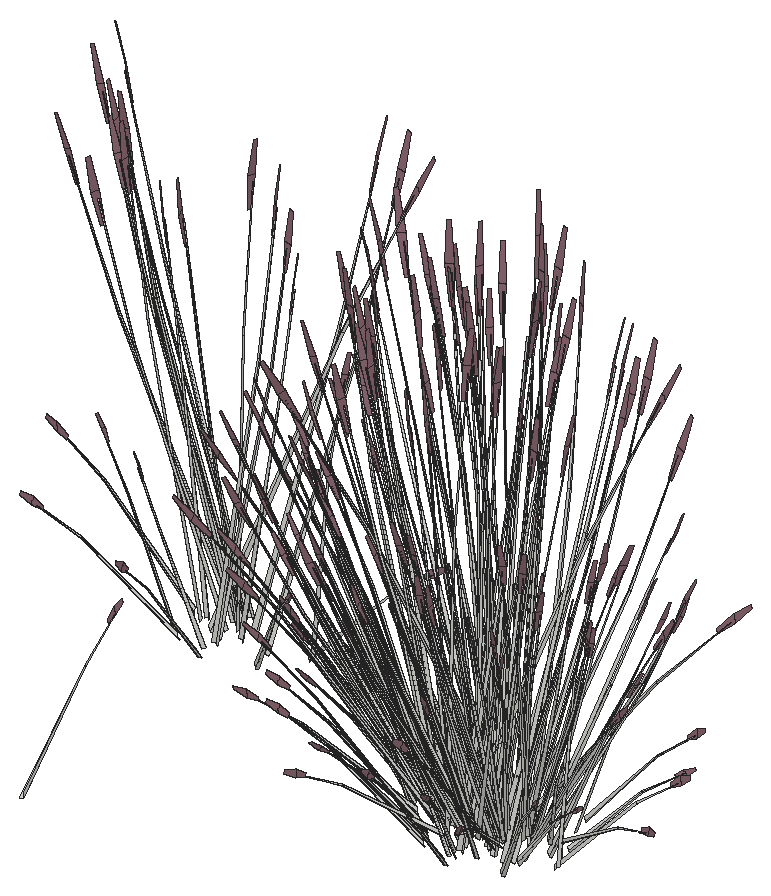
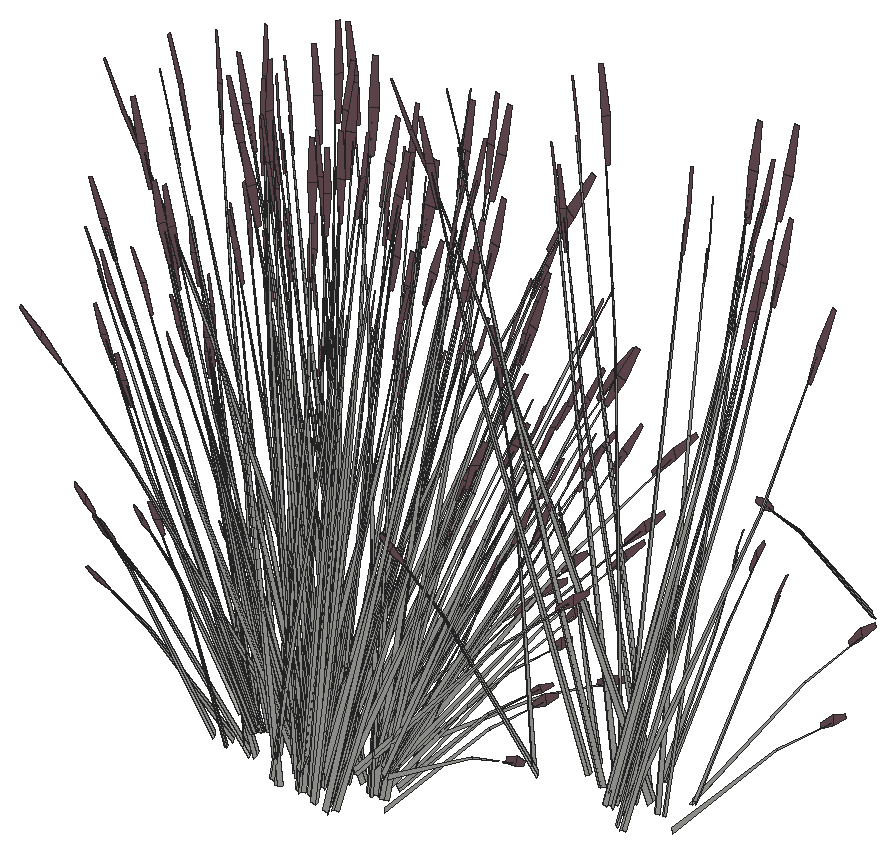
# SketchUp Ruby script. Lengths in inches.
U = 1.inch
M = Sketchup.active_model
def pt(a) = Geom::Point3d.new(a.map { |v| v * U })
def face(e, loops, mat)
  f = e.add_face(loops[0].map { |a| pt(a) })
  loops[1..].each { |l| e.add_face(l.map { |a| pt(a) }).erase! }
  f.material = f.back_material = mat if mat
  f
end
# faces: each face lists its corners as indices into pts; further lists are holes
def faces(e, pts, list, mat = nil) = list.each { |f| face(e, (f[0].is_a?(Array) ? f : [f]).map { |l| l.map { |i| pts[i] } }, mat) }
# xy, xz, yz: faces in a plane at the given z, y or x. An outline is a flat list of corners, or four numbers for a rectangle; further outlines are holes
def ring(l) = l.size == 4 ? [[l[0], l[1]], [l[2], l[1]], [l[2], l[3]], [l[0], l[3]]] : l.each_slice(2).to_a
def flat(e, list, mat, &to3) = list.each { |f| face(e, (f[0].is_a?(Array) ? f : [f]).map { |l| ring(l).map { |u, v| to3.(u, v) } }, mat) }
def xy(e, z, list, mat = nil) = flat(e, list, mat) { |x, y| [x, y, z] }
def xz(e, y, list, mat = nil) = flat(e, list, mat) { |x, z| [x, y, z] }
def yz(e, x, list, mat = nil) = flat(e, list, mat) { |y, z| [x, y, z] }
def lines(e, pts, list) = list.each { |a, b| e.add_line(pt(pts[a]), pt(pts[b])) }
# prism: a flat outline (further loops are holes) pulled along v
def prism(e, loops, v, mat = nil)
  f = face(e, loops, mat); d = Geom::Vector3d.new(v.map { |x| x * U })
  f.pushpull(f.normal.samedirection?(d) ? d.length : -d.length)
end
def box(e, o, s, mat = nil) = prism(e, [[o, [o[0] + s[0], o[1], o[2]], [o[0] + s[0], o[1] + s[1], o[2]], [o[0], o[1] + s[1], o[2]]]], [0, 0, s[2]], mat)
def at(x, y, z, deg = 0) = Geom::Transformation.translation(pt([x, y, z])) * Geom::Transformation.rotation(ORIGIN, Z_AXIS, deg.degrees)
def axes(o, x, y, z) = Geom::Transformation.new([*x, 0, *y, 0, *z, 0, *pt(o).to_a, 1])
def part(name) = M.definitions.add(name)
# library, detail: a bought-in or finely detailed component or shape, given as its bounding box
def library(name, o, s) = part(name).tap { |d| box(d.entities, o, s) }
def detail(e, o, s) = box(e.add_group.entities, o, s)
def put(e, d, t, mat = nil) = e.add_instance(d, t).tap { |i| i.material = mat if mat }
def group(e, t, mat = nil) = e.add_group.tap { |g| g.transformation = t; g.material = mat if mat }.entities
root = M.entities
M.materials.add("LightPink_Translucent").color = [144, 107, 117]
c1 = part("blade")
p = [[2.15,0.21,22],[0,0.17,0],[0.09,0.45,0],[2.18,0.31,22],[2.29,0.31,22],[0.38,0.45,0],
  [2.48,0.24,33],[2.49,0.24,33],[2.48,0.22,33]]
faces(c1.entities,p,[[0,1,2,3],[4,5,2,3],[6,3,4,7],[8,0,3,6]])
c2 = part("seeds")
p = [[0.3,-0.1,1.38],[-0.01,-0.03,1.59],[-0.01,-0.03,0.03],[0.14,-0.07,-0.07],[0.29,-0.03,3],[0.15,0.01,3.11]]
faces(c2.entities,p,[[0,1,2,3],[1,0,4,5]],"LightPink_Translucent")
c3 = part("blade with seeds")
put(c3.entities,c1,at(0,0,0))
put(c3.entities,c2,axes([2.4,0.25,30.99],[1.5799,-0.05474,1.17369],[-0.12525,1.92788,0.29478],[-0.07173,-0.02425,1.56792]))
put(root,c3,axes([47.84,476.29,43.49],[0.19833,-0.05635,1.76342],[1.19302,0.31018,-0.26939],[0.03489,0.3496,0.30037]))
put(root,c3,axes([72.59,505.67,36.13],[0.28013,0.33252,1.71376],[-1.29445,0.27994,0.13857],[-0.29256,-0.52202,0.73262]))
put(root,c3,axes([74.73,503.46,36.97],[-0.18744,-0.14521,1.74944],[-1.25089,0.09206,-0.27667],[-0.19964,-0.34731,0.14031]))
put(root,c3,axes([77.625,505.1875,34.85],[-0.34835,0.20963,1.43002],[-1.04325,-0.36691,-0.30754],[0.19338,-0.4563,0.61141]))
put(root,c3,axes([76.04,505.92,37.24],[-0.5849,-0.8421,-0.71045],[1.20401,-0.4693,0.08574],[-0.13677,-0.40688,1.00501]))
put(root,c3,axes([72.23,504.79,34.85],[-0.07421,0.33879,1.43002],[-1.08488,0.28361,-0.30754],[-0.25359,-0.4379,0.61141]))
put(root,c3,axes([75.03,504.05,33.75],[-0.20555,0.03731,1.76342],[-1.13672,-0.42002,-0.26939],[0.01907,-0.35034,0.30037]))
put(root,c3,axes([78.47,506.74,37.24],[0.03189,-0.95798,-0.71045],[1.34277,0.06434,0.08574],[0.14171,-0.40585,1.00501]))
put(root,c3,axes([80.35,505.24,36.97],[-0.01183,-0.20612,1.74944],[-0.99913,-0.59572,-0.27667],[0.15447,-0.36112,0.14031]))
put(root,c3,axes([76.15,505.2,36.78],[0.36946,-0.79643,-0.35414],[1.07787,0.23229,0.4572],[-0.09883,-0.32066,0.87481]))
put(root,c3,axes([76.96,506.25,36.13],[-0.22818,0.35597,1.71376],[-0.95725,-0.73667,0.13857],[0.43183,-0.45914,0.73262]))
put(root,c3,axes([80.08,504.5,36.96],[-0.12446,0.07911,1.77383],[-1.21937,-0.26689,-0.16761],[-0.04414,-0.34521,0.31391]))
put(root,c3,axes([75.6,505.75,36.94],[-1.20468,-0.25962,-0.51099],[0.41292,-0.89013,-0.3958],[-0.11046,-0.35838,0.97773]))
put(root,c3,axes([76.34,503.52,35.02],[0.15721,0.60392,1.1486],[-0.87211,-0.33448,0.84392],[0.09385,-0.30923,0.25299]))
put(root,c3,axes([78.2,506.42,36.94],[-0.87728,-0.69587,-0.51099],[0.92674,-0.60943,-0.3958],[0.13348,-0.35356,0.97773]))
put(root,c3,axes([73.44,502.99,36.96],[-0.02286,0.12414,1.77383],[-1.12758,0.45052,-0.16761],[-0.33182,-0.23029,0.31391]))
put(root,c3,axes([73.2,505.19,37.35],[1.36515,-0.26619,0.53763],[0.23692,1.04421,0.4433],[-0.32106,-0.30775,1.11249]))
put(root,c3,axes([76.28,505.39,36.99],[1.20755,0.27075,0.48003],[-0.41292,0.89013,0.3958],[-0.07257,-0.35005,0.9933]))
put(root,c3,axes([76.63,505.7,37.29],[-1.19922,0.48218,-0.1216],[-0.58932,-0.85579,-0.67495],[-0.15822,-0.36063,1.02557]))
put(root,c3,axes([79.12,506.79,37.29],[-1.34686,-0.05131,-0.1216],[0.03681,-0.97156,-0.67495],[0.09356,-0.37418,1.02557]))
put(root,c3,axes([79.03,506.16,36.78],[0.82919,-0.54528,-0.35414],[0.78493,0.62262,0.4572],[0.11943,-0.31634,0.87481]))
put(root,c3,axes([71.86,504.24,35.02],[0.63926,0.36046,1.1486],[-0.93099,0.21668,0.84392],[-0.1992,-0.27702,0.25299]))
put(root,c3,axes([76.6,505.32,36.98],[0.90301,-0.35198,0.0643],[0.44199,0.64184,0.50621],[-0.08721,-0.28293,0.77189]))
put(root,c3,axes([73.4,506.15,37.24],[-1.04497,-0.50058,-0.71045],[0.74264,-0.8772,0.08574],[-0.3786,-0.29889,1.00501]))
put(root,c3,axes([73.04,505.49,36.78],[-0.18927,-0.83419,-0.35414],[1.08199,-0.22027,0.4572],[-0.29062,-0.23905,0.87481]))
put(root,c3,axes([45.08,506.35,43.49],[-0.20555,0.03731,1.76342],[-1.13672,-0.42002,-0.26939],[0.01907,-0.35034,0.30037]))
put(root,c3,axes([73.51,505.42,36.98],[0.55698,-0.6579,0.0643],[0.79316,0.38303,0.50621],[-0.25643,-0.21093,0.77189]))
put(root,c3,axes([71.35,505.33,33.75],[-0.11871,0.13643,1.76342],[-1.19964,0.29415,-0.26939],[-0.2898,-0.26759,0.30037]))
put(root,c3,axes([73.33,509.08,34.35],[-0.50328,-1.06202,-0.69835],[1.44974,-0.38248,-0.18329],[-0.05563,-0.35963,1.54149]))
put(root,c3,axes([70.71,506.71,36.13],[0.45521,0.17844,1.71376],[-0.94204,0.74856,0.13857],[-0.58713,-0.33769,0.73262]))
put(root,c3,axes([80.0625,505.83,33.75],[-0.18342,-0.08159,1.76342],[-0.47115,-0.9115,-0.26939],[0.31784,-0.24736,0.30037]))
put(root,c3,axes([76.27,506.04,37.31],[-0.36946,0.79643,0.35414],[-1.07787,-0.23229,-0.4572],[-0.09883,-0.32066,0.87481]))
put(root,c3,axes([72.91,506.18,36.94],[-1.20928,0.24619,-0.51099],[-0.21154,-0.93233,-0.3958],[-0.32481,-0.26718,0.97773]))
put(root,c3,axes([79.02,506.375,36.99],[0.87265,0.70663,0.48003],[-0.92674,0.60943,0.3958],[0.16097,-0.33153,0.9933]))
put(root,c3,axes([73.76,505.35,37.68],[-0.81789,0.99285,-0.13619],[-1.18445,-0.572,-0.75594],[-0.41173,-0.28051,1.14864]))
put(root,c3,axes([79.35,506.44,36.98],[1.00708,0.04826,0.0643],[-0.02761,0.72867,0.50621],[0.10538,-0.27912,0.77189]))
put(root,c3,axes([78.59,506.9375,37.31],[-0.82919,0.54528,0.35414],[-0.78493,-0.62262,-0.4572],[0.11943,-0.31634,0.87481]))
put(root,c3,axes([80.06,508.41,37.24],[0.64013,-0.81717,-0.71045],[1.12174,0.58074,0.08574],[0.38221,-0.29607,1.00501]))
put(root,c3,axes([73.14,506.03,34.63],[-0.7662,-1.03778,0],[1.28187,-0.57875,-0.51607],[0.29196,-0.13181,1.63711]))
put(root,c3,axes([80.02,508.02,36.94],[-0.31482,-0.94565,-0.51099],[1.19224,-0.16542,-0.3958],[0.34166,-0.254,0.97773]))
put(root,c3,axes([74.82,504.78,34.38],[-0.84686,0.59414,-0.03893],[-0.77596,-0.65071,-0.17649],[-0.05463,-0.18438,0.58215]))
put(root,c3,axes([70.625,505.0625,36.97],[-0.26368,-0.00731,1.74944],[-0.83946,0.73103,-0.27667],[-0.44791,-0.14937,0.14031]))
put(root,c3,axes([80.59,508.7,37.29],[-1.1336,-0.57106,-0.1216],[0.65308,-0.827,-0.67495],[0.32027,-0.28747,1.02557]))
put(root,c3,axes([75.9,511.82,35.58],[1.05902,0.41762,1.51261],[-1.03748,0.89969,0.59816],[-0.46471,-0.53324,1.26806]))
put(root,c3,axes([41.41,507.64,43.49],[-0.11871,0.13643,1.76342],[-1.19964,0.29415,-0.26939],[-0.2898,-0.26759,0.30037]))
put(root,c3,axes([73.68,506.17,37.31],[0.18927,0.83419,0.35414],[-1.08199,0.22027,-0.4572],[-0.29062,-0.23905,0.87481]))
put(root,c3,axes([70.37,508.93,34.27],[0,-1.03566,-0.49651],[1.37109,0,0],[0,-0.23588,1.57504]))
put(root,c3,axes([74.18,505.86,34.27],[1.14694,-0.51783,-0.49651],[0.68554,0.92854,0],[0.26122,-0.11794,1.57504]))
put(root,c3,axes([80.98,507.65,34.85],[-0.4378,-0.03068,1.43002],[-0.44851,-0.8229,-0.30754],[0.53783,-0.23279,0.61141]))
put(root,c3,axes([70.43,506.72,37.35],[1.01205,-0.7643,0.53763],[0.87284,0.81167,0.4433],[-0.47482,-0.14098,1.11249]))
put(root,c3,axes([83.38,508.45,36.96],[-0.16006,-0.00787,1.77383],[-0.66468,-0.8428,-0.16761],[0.26693,-0.27711,0.31391]))
put(root,c3,axes([43.39,511.39,44.1],[-0.50328,-1.06202,-0.69835],[1.44974,-0.38248,-0.18329],[-0.05563,-0.35963,1.54149]))
put(root,c3,axes([50.11,508.14,43.49],[-0.18342,-0.08159,1.76342],[-0.47115,-0.9115,-0.26939],[0.31784,-0.24736,0.30037]))
put(root,c3,axes([75.54,507.99,34.3125],[0.82544,-0.77843,-0.62353],[1.0254,0.70586,-0.16365],[0.33076,-0.19418,1.37633]))
put(root,c3,axes([81.49,506.14,35.02],[-0.40819,0.5272,1.1486],[-0.35086,-0.70831,0.84392],[0.33713,-0.17749,0.25299]))
put(root,c3,axes([80.9,508.12,36.78],[1.06674,-0.14801,-0.35414],[0.28168,0.84611,0.4572],[0.30569,-0.22726,0.87481]))
put(root,c3,axes([70.89,506.71,36.98],[0.06171,-0.78753,0.0643],[0.9318,0.02159,0.50621],[-0.35694,-0.08241,0.77189]))
put(root,c3,axes([74.1,509.35,34.47],[0.59459,-0.93321,-0.44739],[1.23546,0.44912,0.21531],[0,-0.21512,1.43643]))
put(root,c3,axes([70.54,506.96,36.78],[-0.69728,-0.64842,-0.35414],[0.79619,-0.61382,0.4572],[-0.40453,-0.09339,0.87481]))
put(root,c3,axes([74.64,508.89,34.92],[-0.1428,-1.18174,-0.29095],[1.48733,-0.07145,-0.50002],[0.26191,-0.15741,1.59708]))
put(root,c3,axes([70.95,508.95,34.28],[0.85545,-0.64616,-0.30978],[0.85545,0.64616,0.30978],[0,-0.20813,1.38974]))
put(root,c3,axes([44.87,507.08,44.13],[-0.84686,0.59414,-0.03893],[-0.77596,-0.65071,-0.17649],[-0.05463,-0.18438,0.58215]))
put(root,c3,axes([70.61,505.86,34.38],[-0.35352,0.84566,-0.03893],[-1.08806,-0.26014,-0.17649],[-0.1652,-0.13832,0.58215]))
put(root,c3,axes([80.03,508.62,37.31],[-1.06674,0.14801,0.35414],[-0.28168,-0.84611,-0.4572],[0.30569,-0.22726,0.87481]))
put(root,c3,axes([73.95,510.13,34.92],[-1.38012,-0.49416,-0.29095],[0.66454,-1.04299,-0.50002],[-0.04337,-0.25608,1.59708]))
put(root,c3,axes([70.02,509.72,34.63],[-1.53239,0,0],[0,-1.1575,-0.51607],[0,-0.26363,1.63711]))
put(root,c3,axes([70.29,507.65,34.85],[0.23927,0.28834,1.43002],[-0.55135,0.78376,-0.30754],[-0.56612,-0.18733,0.61141]))
put(root,c3,axes([74.45,506.27,34.28],[1.14332,0.25625,-0.30978],[-0.28787,0.90242,0.30978],[0.23049,-0.10406,1.38974]))
put(root,c3,axes([71.27,507.39,37.24],[-1.22504,-0.02494,-0.71045],[0.08228,-1.05005,0.08574],[-0.51899,-0.11081,1.00501]))
put(root,c3,axes([40.42,511.24,44.02],[0,-1.03566,-0.49651],[1.37109,0,0],[0,-0.23588,1.57504]))
put(root,c3,axes([44.23,508.17,44.02],[1.14694,-0.51783,-0.49651],[0.68554,0.92854,0],[0.26122,-0.11794,1.57504]))
put(root,c3,axes([81,508.49,36.98],[0.8413,0.43556,0.0643],[-0.48981,0.62025,0.50621],[0.26973,-0.20053,0.77189]))
put(root,c3,axes([80.77,508.31,36.99],[0.30393,0.95317,0.48003],[-1.19224,0.16542,0.3958],[0.35138,-0.22417,0.9933]))
put(root,c3,axes([83.98,509.46,36.97],[0.17006,-0.15775,1.74944],[-0.21766,-0.96766,-0.27667],[0.42669,-0.18347,0.14031]))
put(root,c3,axes([45.59,510.3,44.06],[0.82544,-0.77843,-0.62353],[1.0254,0.70586,-0.16365],[0.33076,-0.19418,1.37633]))
put(root,c3,axes([71.21,509.41,34.58],[-1.1399,0.87071,0.30756],[-1.1406,-0.86155,-0.36492],[-0.03981,-0.24727,1.64885]))
put(root,c3,axes([69.61,505.68,36.96],[0.09085,0.10335,1.77383],[-0.43798,0.92907,-0.16761],[-0.44357,0.00672,0.31391]))
put(root,c3,axes([74.84,509.82,34.6875],[1.3808,0.50196,0.24065],[-0.66454,1.04299,0.50002],[0,-0.24043,1.60543]))
put(root,c3,axes([74.3,511.23,34.69],[0.32481,-1.2272,-0.23429],[1.54007,0.21392,0.51271],[-0.26911,-0.16947,1.5644]))
put(root,c3,axes([44.15,511.66,44.21],[0.59459,-0.93321,-0.44739],[1.23546,0.44912,0.21531],[0,-0.21512,1.43643]))
put(root,c3,axes([70.87,507.6,36.94],[-0.88986,0.68603,-0.51099],[-0.77932,-0.72471,-0.3958],[-0.45212,-0.10438,0.97773]))
put(root,c3,axes([44.69,511.2,44.67],[-0.1428,-1.18174,-0.29095],[1.48733,-0.07145,-0.50002],[0.26191,-0.15741,1.59708]))
put(root,c3,axes([71.53,507.3,37.31],[0.69728,0.64842,0.35414],[-0.79619,0.61382,-0.4572],[-0.40453,-0.09339,0.87481]))
put(root,c3,axes([41.01,511.26,44.03],[0.85545,-0.64616,-0.30978],[0.85545,0.64616,0.30978],[0,-0.20813,1.38974]))
put(root,c3,axes([68.86,508.51,35.02],[0.78239,-0.07411,1.1486],[-0.49629,0.65296,0.84392],[-0.38663,-0.09795,0.25299]))
put(root,c3,axes([40.66,508.16,44.13],[-0.35352,0.84566,-0.03893],[-1.08806,-0.26014,-0.17649],[-0.1652,-0.13832,0.58215]))
put(root,c3,axes([44,512.4375,44.67],[-1.38012,-0.49416,-0.29095],[0.66454,-1.04299,-0.50002],[-0.04337,-0.25608,1.59708]))
put(root,c3,axes([74.39,509.12,34.97],[-1.33077,0.06393,0.44739],[-0.12035,-1.06125,-0.21531],[0.23824,-0.10756,1.43643]))
put(root,c3,axes([71.33,506.89,37.29],[-0.06562,1.05324,-0.1216],[-1.2424,-0.02879,-0.67495],[-0.4785,-0.07316,1.02557]))
put(root,c3,axes([70.95,509.89,34.73],[0,1.03566,0.49651],[-1.37109,0,0],[0,-0.23588,1.57504]))
put(root,c3,axes([80.63,510.93,37.29],[-0.6166,-0.93779,-0.1216],[1.09436,-0.46085,-0.67495],[0.46117,-0.12373,1.02557]))
put(root,c3,axes([44.5,508.58,44.03],[1.14332,0.25625,-0.30978],[-0.28787,0.90242,0.30978],[0.23049,-0.10406,1.38974]))
put(root,c3,axes([80.58,510.12,36.94],[0.332,-0.94205,-0.51099],[1.13828,0.3229,-0.3958],[0.45829,-0.08638,0.97773]))
put(root,c3,axes([78.78,506.29,34.63],[0.7662,-1.03778,0],[1.28187,0.57875,-0.51607],[0.29196,0.13181,1.63711]))
put(root,c3,axes([69.75,508.34,36.13],[0.50831,-0.02346,1.71376],[-0.33721,1.01661,0.13857],[-0.72439,-0.06288,0.73262]))
put(root,c3,axes([74.19,510.73,34.47],[-0.73619,-0.86927,-0.44739],[1.11511,-0.61213,0.21531],[-0.23824,-0.10756,1.43643]))
put(root,c3,axes([74.34,509.5,34.62],[0.53281,1.15808,0.45755],[-1.52239,0.4027,0.17955],[0.01861,-0.2128,1.58856]))
put(root,c3,axes([81.79,510.39,34.24],[-0.7893,0.12429,1.41583],[-0.12563,-0.9893,0.08104],[0.55282,-0.14974,0.80566]))
put(root,c3,axes([83.23,509.51,34.52],[-0.75977,-0.66224,-0.06488],[0.83212,-0.6068,-0.29416],[0.23578,-0.04272,0.97024]))
put(root,c3,axes([74.08,510.41,34.97],[-0.59459,0.93321,0.44739],[-1.23546,-0.44912,-0.21531],[0,-0.21512,1.43643]))
put(root,c3,axes([76.26,509.6,34.46],[0,-1.19833,0],[1.53239,0,0],[0,0,1.79456]))
put(root,c3,axes([78.12,506.83,34.73],[-1.14694,-0.51783,0.49651],[0.68554,-0.92854,0],[0.26122,0.11794,1.57504]))
put(root,c3,axes([80.36,510.47,37.24],[1.07686,-0.45739,-0.71045],[0.60013,0.94154,0.08574],[0.52031,-0.10696,1.00501]))
put(root,c3,axes([73.53,511.0625,34.3125],[-1.27479,-0.1698,-0.62353],[0.26901,-1.04736,-0.16365],[-0.38043,-0.12691,1.37633]))
put(root,c3,axes([75.53,508.84,34.62],[-1.01611,0.93987,0.45755],[-1.20717,-0.82966,0.17955],[0.24496,-0.0938,1.58856]))
put(root,c3,axes([76.64,510.53,34.55],[-1.1399,-0.8914,-0.06131],[1.1406,-0.89194,0],[-0.03981,-0.03113,1.75571]))
put(root,c3,axes([73.77,507.3,34.73],[-0.35402,1.02926,0.17642],[-1.29548,-0.29127,0.35086],[0.22379,-0.00501,1.60407]))
put(root,c3,axes([80.2,510.65,37.31],[-1.01846,-0.28891,0.35414],[0.29705,-0.84289,-0.4572],[0.41005,-0.07729,0.87481]))
put(root,c3,axes([44.35,513.53,44.4375],[0.32481,-1.2272,-0.23429],[1.54007,0.21392,0.51271],[-0.26911,-0.16947,1.5644]))
put(root,c3,axes([69.54,509.11,36.99],[0.34623,-0.9443,0.48003],[1.13828,0.3229,0.3958],[-0.44763,0.05675,0.9933]))
put(root,c3,axes([73.23,508.125,33.85],[-1.20625,0.41464,1.28929],[-0.38394,-1.1897,0.50096],[0.74071,0.01979,1.46642]))
put(root,c3,axes([76.48,508.44,34.87],[0.23642,-0.92427,0.1448],[1.15506,0.16044,-0.41347],[0.21021,0.09491,1.26744]))
put(root,c3,axes([69.46,508.86,36.98],[-0.4501,-0.70615,0.0643],[0.82077,-0.34564,0.50621],[-0.36181,0.0682,0.77189]))
put(root,c3,axes([74.48,510.64,34.62],[1.54892,0.2182,0.45755],[-0.31522,1.23236,0.17955],[-0.22636,-0.119,1.58856]))
put(root,c3,axes([82.66,509.74,33.75],[-0.06405,-0.15723,1.76342],[0.44421,-0.91974,-0.26939],[0.4481,-0.01323,0.30037]))
put(root,c3,axes([69.43,509.58,33.75],[0.03108,0.16322,1.76342],[-0.62654,0.85237,-0.26939],[-0.44504,-0.04296,0.30037]))
put(root,c3,axes([75.98,508.68,34.97],[-0.73619,-0.86927,0.44739],[1.11511,-0.61213,-0.21531],[0.23824,0.10756,1.43643]))
put(root,c3,axes([72.18,512.66,34.28],[-0.28787,-0.90242,-0.30978],[1.14332,-0.25625,0.30978],[-0.23049,-0.10406,1.38974]))
put(root,c3,axes([44.24,513.03,44.21],[-0.73619,-0.86927,-0.44739],[1.11511,-0.61213,0.21531],[-0.23824,-0.10756,1.43643]))
put(root,c3,axes([73.65,512.6,34.73],[1.31687,-0.27488,0.17642],[0.32517,1.02297,0.35086],[-0.11745,-0.14905,1.60407]))
put(root,c3,axes([76.36,508.74,34.92],[1.23732,-0.68758,-0.29095],[0.8228,0.97154,-0.50002],[0.30528,0.09867,1.59708]))
put(root,c3,axes([81.28,510.55,36.78],[1.01846,0.28891,-0.35414],[-0.29705,0.84289,0.4572],[0.41005,-0.07729,0.87481]))
put(root,c3,axes([53.28,511.82,44.26],[-0.75977,-0.66224,-0.06488],[0.83212,-0.6068,-0.29416],[0.23578,-0.04272,0.97024]))
put(root,c3,axes([71.86,513.04,34.27],[-1.14694,-0.51783,-0.49651],[0.68554,-0.92854,0],[-0.26122,-0.11794,1.57504]))
put(root,c3,axes([79.48,506.91,34.27],[1.14694,0.51783,-0.49651],[-0.68554,0.92854,0],[0.26122,0.11794,1.57504]))
put(root,c3,axes([69.31,509.21,36.78],[-1.01846,-0.28891,-0.35414],[0.29705,-0.84289,0.4572],[-0.41005,0.07729,0.87481]))
put(root,c3,axes([77.3,509.87,34.46],[1.37109,0,0],[0,1.07219,0],[0,0,1.78407]))
put(root,c3,axes([74.98,511.22,34.92],[-1.23732,0.68758,-0.29095],[-0.8228,-0.97154,-0.50002],[-0.30528,-0.09867,1.59708]))
put(root,c3,axes([77.6875,507.35,34.73],[-1.31687,0.27488,0.17642],[-0.32517,-1.02297,0.35086],[0.11745,0.14905,1.60407]))
put(root,c3,axes([78.5,509.51,36.13],[-0.50831,0.02346,1.71376],[0.33721,-1.01661,0.13857],[0.72439,0.06288,0.73262]))
put(root,c3,axes([79.16,507.3,34.28],[0.28787,0.90242,-0.30978],[-1.14332,0.25625,0.30978],[0.23049,0.10406,1.38974]))
put(root,c3,axes([43.58,513.37,44.06],[-1.27479,-0.1698,-0.62353],[0.26901,-1.04736,-0.16365],[-0.38043,-0.12691,1.37633]))
put(root,c3,axes([81.125,510.91,36.98],[0.4501,0.70615,0.0643],[-0.82077,0.34564,0.50621],[0.36181,-0.0682,0.77189]))
put(root,c3,axes([76.86,509.32,34.64],[-1.54892,-0.2182,0.49198],[0.31522,-1.23236,0.19306],[0.22636,0.119,1.70813]))
put(root,c3,axes([81.04,510.66,36.99],[-0.34623,0.9443,0.48003],[-1.13828,-0.3229,0.3958],[0.44763,-0.05675,0.9933]))
put(root,c3,axes([75.62,512.36,34.46],[-0.39985,-0.89288,0],[1.1418,-0.31268,0],[0,0,1.54371]))
put(root,c3,axes([74.86,511.52,34.87],[-0.23642,0.92427,0.1448],[-1.15506,-0.16044,-0.41347],[-0.21021,-0.09491,1.26744]))
put(root,c3,axes([70.38,509.12,37.31],[1.01846,0.28891,0.35414],[-0.29705,0.84289,-0.4572],[-0.41005,0.07729,0.87481]))
put(root,c3,axes([43.29,510.43,43.59],[-1.20625,0.41464,1.28929],[-0.38394,-1.1897,0.50096],[0.74071,0.01979,1.46642]))
put(root,c3,axes([77.12,512.24,34.4375],[1.2866,-0.3514,-0.19198],[0.45209,1.01223,0.00008],[0.14202,-0.03884,1.73897]))
put(root,c3,axes([77.5625,512.66,34.73],[0.35402,-1.02926,0.17642],[1.29548,0.29127,0.35086],[-0.22379,0.00501,1.60407]))
put(root,c3,axes([52.71,512.05,43.49],[-0.06405,-0.15723,1.76342],[0.44421,-0.91974,-0.26939],[0.4481,-0.01323,0.30037]))
put(root,c3,axes([77.27,510.33,34.47],[0.85545,0.66896,0],[-0.85545,0.66896,0],[0,0,1.69266]))
put(root,c3,axes([39.48,511.89,43.49],[0.03108,0.16322,1.76342],[-0.62654,0.85237,-0.26939],[-0.44504,-0.04296,0.30037]))
put(root,c3,axes([72.41,509.07,35.6],[0.34834,-0.14982,1.77064],[0.12012,1.04605,0.13857],[-0.75452,0.1388,0.63284]))
put(root,c3,axes([79.59,510.03,34.73],[-0.96285,-0.75439,0.17642],[0.97031,-0.7317,0.35086],[-0.10634,0.15406,1.60407]))
put(root,c3,axes([77.8,508.89,34.3125],[1.27479,0.1698,-0.62353],[-0.26901,1.04736,-0.16365],[0.38043,0.12691,1.37633]))
put(root,c3,axes([83.4375,510.72,35.02],[-0.75718,0.17097,1.1486],[0.35641,-0.70661,0.84392],[0.40168,0.04835,0.25299]))
put(root,c3,axes([42.23,514.96,44.03],[-0.28787,-0.90242,-0.30978],[1.14332,-0.25625,0.30978],[-0.23049,-0.10406,1.38974]))
put(root,c3,axes([75.34,512.77,34.45],[-1.23546,-0.46496,0],[0.59459,-0.96613,0],[0,0,1.62707]))
put(root,c3,axes([76.37,511.53,34.72],[-1.19666,-0.83357,-0.25192],[1.00694,-0.93603,0.5513],[-0.32224,0.09751,1.68216]))
put(root,c3,axes([73.22,513.125,34.73],[1.14694,0.51783,0.49651],[-0.68554,0.92854,0],[-0.26122,-0.11794,1.57504]))
put(root,c3,axes([46.41,511.05,44.67],[1.23732,-0.68758,-0.29095],[0.8228,0.97154,-0.50002],[0.30528,0.09867,1.59708]))
put(root,c3,axes([77.26,509.54,34.97],[0.59459,-0.93321,0.44739],[1.23546,0.44912,-0.21531],[0,0.21512,1.43643]))
put(root,c3,axes([83.08,513.71,36.96],[-0.11081,-0.09067,1.77383],[0.2424,-0.97188,-0.16761],[0.43649,-0.06209,0.31391]))
put(root,c3,axes([41.91,515.35,44.02],[-1.14694,-0.51783,-0.49651],[0.68554,-0.92854,0],[-0.26122,-0.11794,1.57504]))
put(root,c3,axes([49.53,509.22,44.02],[1.14694,0.51783,-0.49651],[-0.68554,0.92854,0],[0.26122,0.11794,1.57504]))
put(root,c3,axes([68.66,509.77,36.97],[-0.20012,0.13446,1.74944],[0.01702,0.98243,-0.27667],[-0.45871,0.12776,0.14031]))
put(root,c3,axes([77.03,510.08,34.55],[0,1.19774,-0.05637],[-1.53239,0,0],[0,0.03764,1.79368]))
put(root,c3,axes([70,509.64,36.94],[-0.332,0.94205,-0.51099],[-1.13828,-0.3229,-0.3958],[-0.45829,0.08638,0.97773]))
put(root,c3,axes([69.95,508.83,37.29],[0.6166,0.93779,-0.1216],[-1.09436,0.46085,-0.67495],[-0.46117,0.12373,1.02557]))
put(root,c3,axes([45.03,513.52,44.67],[-1.23732,0.68758,-0.29095],[-0.8228,-0.97154,-0.50002],[-0.30528,-0.09867,1.59708]))
put(root,c3,axes([77.14,509.23,34.47],[0.73619,0.86927,-0.44739],[-1.11511,0.61213,0.21531],[0.23824,0.10756,1.43643]))
put(root,c3,axes([82.12,512.9,36.18],[-0.23455,-0.87059,-0.03492],[1.10861,-0.20015,-0.15832],[0.23151,0.05519,0.52218]))
put(root,c3,axes([72.56,513.67,34.63],[-0.7662,1.03778,0],[-1.28187,-0.57875,-0.51607],[-0.29196,-0.13181,1.63711]))
